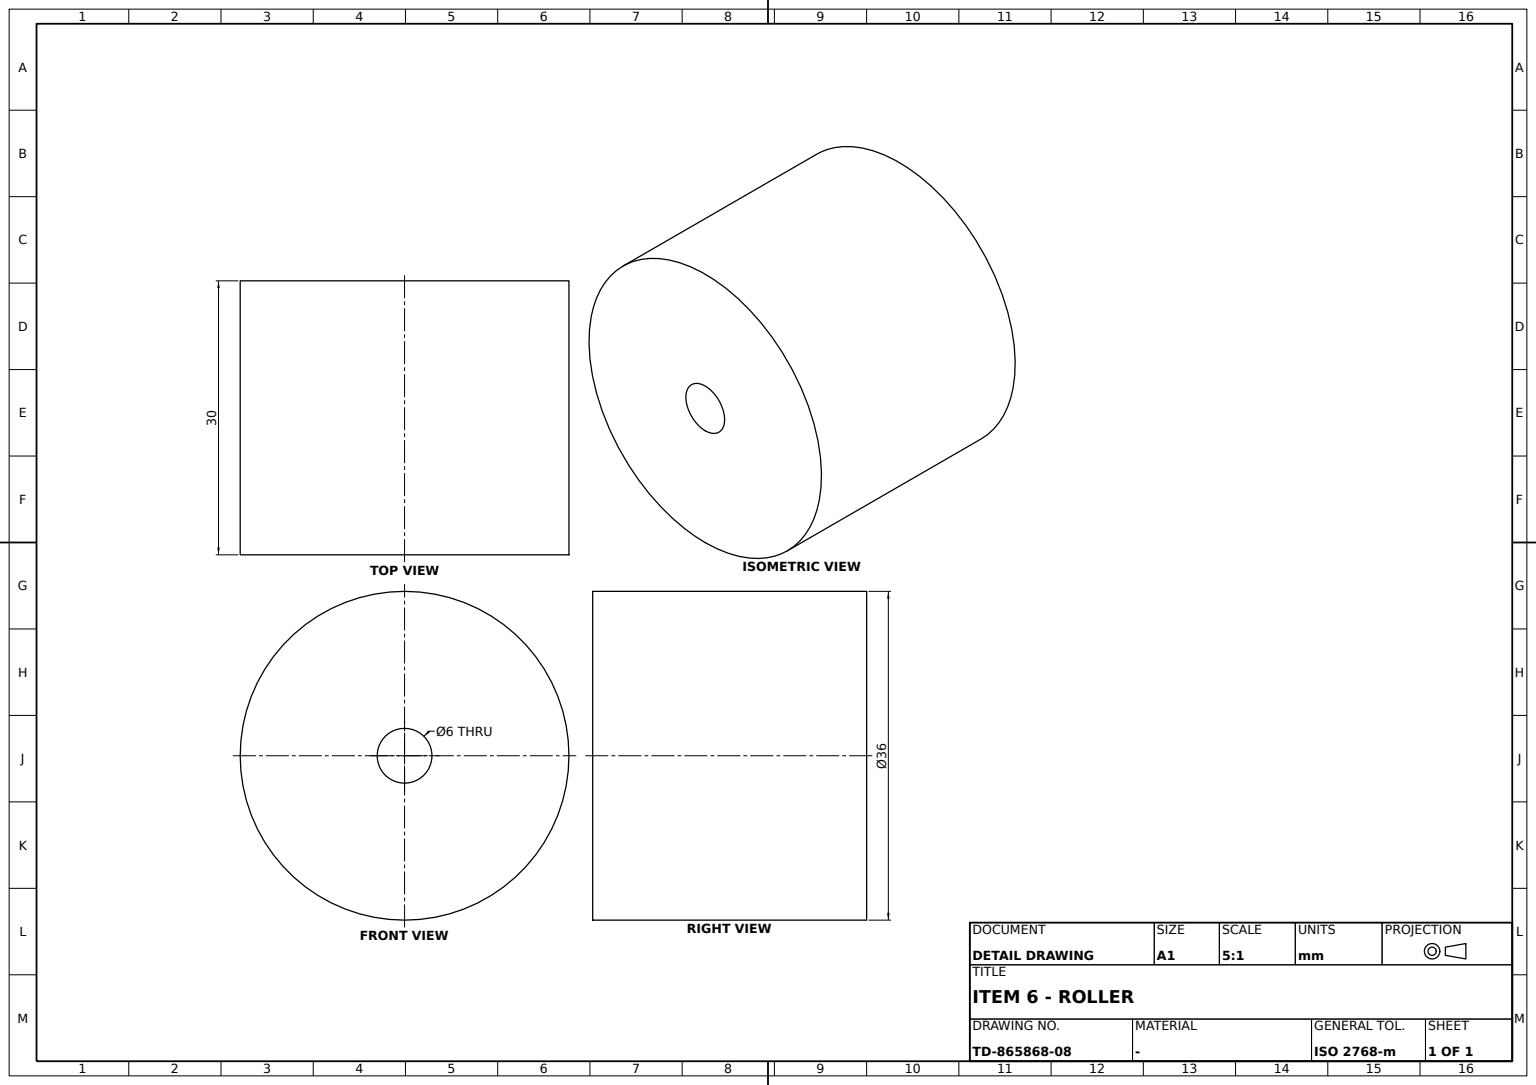
ISO-10303-21;
HEADER;
FILE_DESCRIPTION((''),'2;1');
FILE_NAME('','',(''),(''),'','','');
FILE_SCHEMA(('AUTOMOTIVE_DESIGN'));
ENDSEC;
DATA;
#1=APPLICATION_CONTEXT('');
#2=PRODUCT_CONTEXT('',#1,'mechanical');
#3=PRODUCT('','','',(#2));
#4=PRODUCT_DEFINITION_FORMATION('','',#3);
#5=PRODUCT_DEFINITION_CONTEXT('',#1,'design');
#6=PRODUCT_DEFINITION('','',#4,#5);
#7=PRODUCT_DEFINITION_SHAPE('','',#6);
#8=(LENGTH_UNIT()NAMED_UNIT(*)SI_UNIT(.MILLI.,.METRE.));
#9=(NAMED_UNIT(*)PLANE_ANGLE_UNIT()SI_UNIT($,.RADIAN.));
#10=(NAMED_UNIT(*)SI_UNIT($,.STERADIAN.)SOLID_ANGLE_UNIT());
#11=UNCERTAINTY_MEASURE_WITH_UNIT(LENGTH_MEASURE(0.005),#8,'distance_accuracy_value','');
#12=(GEOMETRIC_REPRESENTATION_CONTEXT(3)GLOBAL_UNCERTAINTY_ASSIGNED_CONTEXT((#11))GLOBAL_UNIT_ASSIGNED_CONTEXT((#8,#9,#10))REPRESENTATION_CONTEXT('',''));
#13=CARTESIAN_POINT('',(15.,0.,-18.));
#14=VERTEX_POINT('',#13);
#15=CARTESIAN_POINT('',(15.,0.,0.));
#16=DIRECTION('',(1.,0.,0.));
#17=DIRECTION('',(0.,0.,-1.));
#18=AXIS2_PLACEMENT_3D('',#15,#16,#17);
#19=CIRCLE('',#18,18.);
#20=EDGE_CURVE('',#14,#14,#19,.T.);
#21=ORIENTED_EDGE('',*,*,#20,.F.);
#22=EDGE_LOOP('',(#21));
#23=FACE_BOUND('',#22,.T.);
#24=CARTESIAN_POINT('',(-15.,0.,-18.));
#25=VERTEX_POINT('',#24);
#26=CARTESIAN_POINT('',(-15.,0.,0.));
#27=AXIS2_PLACEMENT_3D('',#26,#16,#17);
#28=CIRCLE('',#27,18.);
#29=EDGE_CURVE('',#25,#25,#28,.T.);
#30=ORIENTED_EDGE('',*,*,#29,.T.);
#31=EDGE_LOOP('',(#30));
#32=FACE_BOUND('',#31,.T.);
#33=CARTESIAN_POINT('',(0.,0.,0.));
#34=DIRECTION('',(0.,1.,0.));
#35=AXIS2_PLACEMENT_3D('',#33,#16,#34);
#36=CYLINDRICAL_SURFACE('',#35,18.);
#37=ADVANCED_FACE('',(#23,#32),#36,.T.);
#38=CARTESIAN_POINT('',(15.,0.,-3.));
#39=VERTEX_POINT('',#38);
#40=CIRCLE('',#18,3.);
#41=EDGE_CURVE('',#39,#39,#40,.T.);
#42=ORIENTED_EDGE('',*,*,#41,.T.);
#43=EDGE_LOOP('',(#42));
#44=FACE_BOUND('',#43,.T.);
#45=CARTESIAN_POINT('',(-15.,0.,-3.));
#46=VERTEX_POINT('',#45);
#47=CIRCLE('',#27,3.);
#48=EDGE_CURVE('',#46,#46,#47,.T.);
#49=ORIENTED_EDGE('',*,*,#48,.F.);
#50=EDGE_LOOP('',(#49));
#51=FACE_BOUND('',#50,.T.);
#52=CYLINDRICAL_SURFACE('',#35,3.);
#53=ADVANCED_FACE('',(#44,#51),#52,.F.);
#54=ORIENTED_EDGE('',*,*,#41,.F.);
#55=EDGE_LOOP('',(#54));
#56=FACE_BOUND('',#55,.T.);
#57=ORIENTED_EDGE('',*,*,#20,.T.);
#58=EDGE_LOOP('',(#57));
#59=FACE_BOUND('',#58,.T.);
#60=AXIS2_PLACEMENT_3D('',#15,#16,#34);
#61=PLANE('',#60);
#62=ADVANCED_FACE('',(#56,#59),#61,.T.);
#63=ORIENTED_EDGE('',*,*,#29,.F.);
#64=EDGE_LOOP('',(#63));
#65=FACE_BOUND('',#64,.T.);
#66=ORIENTED_EDGE('',*,*,#48,.T.);
#67=EDGE_LOOP('',(#66));
#68=FACE_BOUND('',#67,.T.);
#69=AXIS2_PLACEMENT_3D('',#26,#16,#34);
#70=PLANE('',#69);
#71=ADVANCED_FACE('',(#65,#68),#70,.F.);
#72=CLOSED_SHELL('',(#37,#53,#62,#71));
#73=MANIFOLD_SOLID_BREP('',#72);
#74=ADVANCED_BREP_SHAPE_REPRESENTATION('',(#73),#12);
#75=SHAPE_DEFINITION_REPRESENTATION(#7,#74);
ENDSEC;
END-ISO-10303-21;
